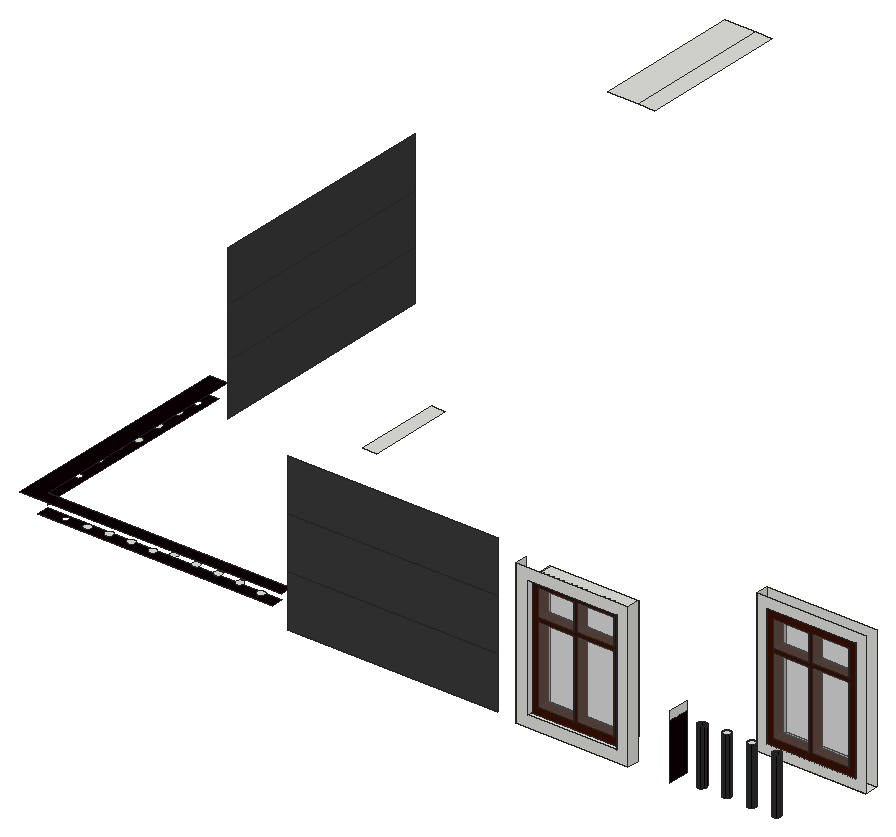
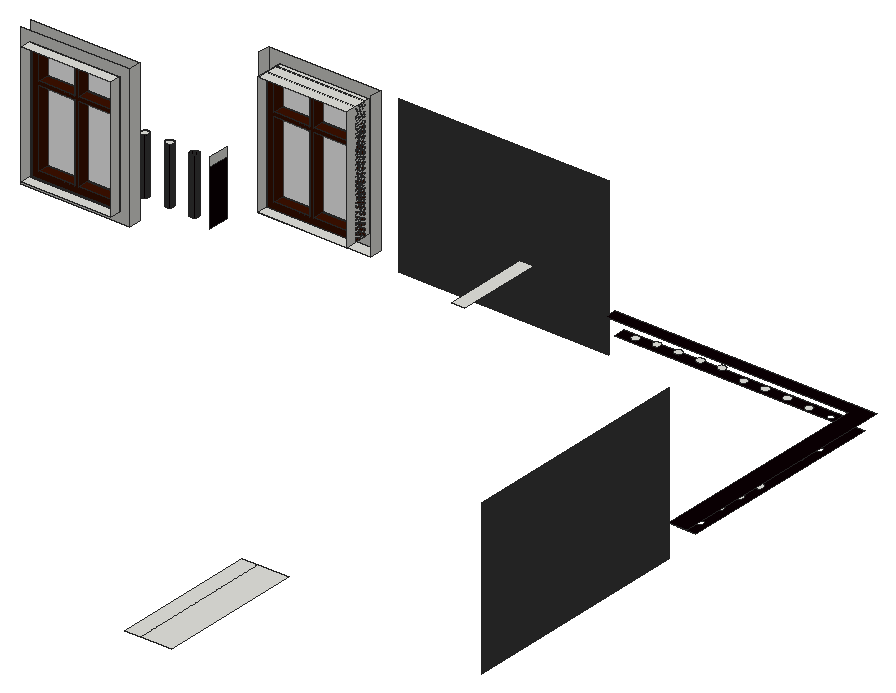
# SketchUp Ruby script. Lengths in inches.
U = 1.inch
M = Sketchup.active_model
def pt(a) = Geom::Point3d.new(a.map { |v| v * U })
def face(e, loops, mat)
  f = e.add_face(loops[0].map { |a| pt(a) })
  loops[1..].each { |l| e.add_face(l.map { |a| pt(a) }).erase! }
  f.material = f.back_material = mat if mat
  f
end
# faces: each face lists its corners as indices into pts; further lists are holes
def faces(e, pts, list, mat = nil) = list.each { |f| face(e, (f[0].is_a?(Array) ? f : [f]).map { |l| l.map { |i| pts[i] } }, mat) }
# xy, xz, yz: faces in a plane at the given z, y or x. An outline is a flat list of corners, or four numbers for a rectangle; further outlines are holes
def ring(l) = l.size == 4 ? [[l[0], l[1]], [l[2], l[1]], [l[2], l[3]], [l[0], l[3]]] : l.each_slice(2).to_a
def flat(e, list, mat, &to3) = list.each { |f| face(e, (f[0].is_a?(Array) ? f : [f]).map { |l| ring(l).map { |u, v| to3.(u, v) } }, mat) }
def xy(e, z, list, mat = nil) = flat(e, list, mat) { |x, y| [x, y, z] }
def xz(e, y, list, mat = nil) = flat(e, list, mat) { |x, z| [x, y, z] }
def yz(e, x, list, mat = nil) = flat(e, list, mat) { |y, z| [x, y, z] }
def lines(e, pts, list) = list.each { |a, b| e.add_line(pt(pts[a]), pt(pts[b])) }
# prism: a flat outline (further loops are holes) pulled along v
def prism(e, loops, v, mat = nil)
  f = face(e, loops, mat); d = Geom::Vector3d.new(v.map { |x| x * U })
  f.pushpull(f.normal.samedirection?(d) ? d.length : -d.length)
end
def box(e, o, s, mat = nil) = prism(e, [[o, [o[0] + s[0], o[1], o[2]], [o[0] + s[0], o[1] + s[1], o[2]], [o[0], o[1] + s[1], o[2]]]], [0, 0, s[2]], mat)
def at(x, y, z, deg = 0) = Geom::Transformation.translation(pt([x, y, z])) * Geom::Transformation.rotation(ORIGIN, Z_AXIS, deg.degrees)
def axes(o, x, y, z) = Geom::Transformation.new([*x, 0, *y, 0, *z, 0, *pt(o).to_a, 1])
def part(name) = M.definitions.add(name)
# library, detail: a bought-in or finely detailed component or shape, given as its bounding box
def library(name, o, s) = part(name).tap { |d| box(d.entities, o, s) }
def detail(e, o, s) = box(e.add_group.entities, o, s)
def put(e, d, t, mat = nil) = e.add_instance(d, t).tap { |i| i.material = mat if mat }
def group(e, t, mat = nil) = e.add_group.tap { |g| g.transformation = t; g.material = mat if mat }.entities
root = M.entities
M.materials.add("[Color C08]").color = [60, 17, 0]
M.materials.add("[Color M07]").color = [58, 58, 58]
M.materials.add("[Metal Seamed]").color = [11, 0, 4]
M.materials.add("[Translucent Glass Gray]").color = [128, 128, 128]
M.materials["[Translucent Glass Gray]"].alpha = 0.5
c1 = part("Group\#3")
xy(c1.entities,0,[[0,0,51.6875,4]],"[Color C08]")
xy(c1.entities,4.05,[[4.05,0,24.41,4],[24.41,0,26.55,4],[26.55,0,47.64,4]],"[Color C08]")
xy(c1.entities,49.59,[[4.05,0,24.41,4],[26.55,0,47.64,4]],"[Color C08]")
xy(c1.entities,51.6875,[[4.05,0,24.41,4],[26.55,0,47.64,4]],"[Color C08]")
xy(c1.entities,67.57,[[4.05,0,24.41,4],[26.55,0,47.64,4]],"[Color C08]")
xy(c1.entities,71.625,[[0,0,51.6875,4]],"[Color C08]")
xz(c1.entities,0,[[[0,0,51.6875,71.625],[4.05,4.05,4.05,49.59,24.41,49.59,24.41,4.05,26.55,4.05,26.55,49.59,47.64,49.59,47.64,4.05],[26.55,51.6875,47.64,67.57],[4.05,51.6875,24.41,67.57]]],"[Color C08]")
xz(c1.entities,0,[[4.05,4.05,24.41,49.59],[26.55,4.05,47.64,49.59],[4.05,51.6875,24.41,67.57],[26.55,51.6875,47.64,67.57]],"[Translucent Glass Gray]")
xz(c1.entities,4,[[[0,0,51.6875,71.625],[4.05,4.05,4.05,49.59,24.41,49.59,24.41,4.05,26.55,4.05,26.55,49.59,47.64,49.59,47.64,4.05],[26.55,51.6875,47.64,67.57],[4.05,51.6875,24.41,67.57]]],"[Color C08]")
yz(c1.entities,0,[[0,0,4,71.625]],"[Color C08]")
yz(c1.entities,4.05,[[0,4.05,4,49.59],[0,51.6875,4,67.57]],"[Color C08]")
yz(c1.entities,24.41,[[0,4.05,4,49.59],[0,51.6875,4,67.57]],"[Color C08]")
yz(c1.entities,26.55,[[0,4.05,4,49.59],[0,51.6875,4,67.57]],"[Color C08]")
yz(c1.entities,47.64,[[0,4.05,4,49.59],[0,51.6875,4,67.57]],"[Color C08]")
yz(c1.entities,51.6875,[[0,0,4,71.625]],"[Color C08]")
xy(root,300,[[382.22,74.99,381.61,75.05,381.05,75.25,380.55,75.6,380.16,76.06,379.91,76.61,379.8,77.2,379.85,77.8,380.06,78.37,380.41,78.86,380.87,79.25,381.41,79.51,382.01,79.61,382.61,79.5625,383.18,79.36,383.67,79.01,384.0625,78.55,384.32,78,384.42,77.41,384.37,76.81,384.16,76.24,383.82,75.74,383.36,75.36,382.81,75.1],[396.15,74.99,395.55,75.05,394.98,75.25,394.49,75.6,394.1,76.06,393.85,76.61,393.74,77.2,393.79,77.8,394,78.37,394.34,78.86,394.81,79.25,395.35,79.51,395.95,79.61,396.55,79.5625,397.12,79.36,397.61,79.01,398,78.55,398.25,78,398.36,77.41,398.31,76.81,398.1,76.24,397.76,75.74,397.29,75.36,396.75,75.1],[410.09,74.99,409.49,75.05,408.92,75.25,408.43,75.6,408.04,76.06,407.78,76.61,407.68,77.2,407.73,77.8,407.94,78.37,408.28,78.86,408.74,79.25,409.29,79.51,409.88,79.61,410.49,79.5625,411.05,79.36,411.55,79.01,411.9375,78.55,412.19,78,412.3,77.41,412.25,76.81,412.04,76.24,411.69,75.74,411.23,75.36,410.69,75.1],[424.03,74.99,423.43,75.05,422.86,75.25,422.36,75.6,421.98,76.06,421.72,76.61,421.61,77.2,421.67,77.8,421.87,78.37,422.22,78.86,422.68,79.25,423.23,79.51,423.82,79.61,424.42,79.5625,424.99,79.36,425.49,79.01,425.875,78.55,426.13,78,426.24,77.41,426.18,76.81,425.98,76.24,425.63,75.74,425.17,75.36,424.62,75.1]])
xy(root,306.73,[[291.14,60.85,353.83,67.28]])
xy(root,307.48,[[389.45,106.41,450.64,113.66]])
xy(root,313.04,[[297.45,60.85,347.52,76.28],[395.02,106.41,445.08,113.66],[395.02,113.66,445.08,119.66]])
xy(root,316.34,[[[21.75,62.76,153.04,69.57],[33.7,65.03,34.2,65.05,34.6875,65.21,35.11,65.48,35.45,65.86,35.68,66.3125,35.78,66.81,35.76,67.3125,35.6,67.79,35.32,68.22,34.95,68.55,34.5,68.78,34,68.89,33.5,68.86,33.02,68.71,32.59,68.43,32.25,68.05,32.02,67.6,31.92,67.11,31.95,66.6,32.1,66.12,32.38,65.7,32.75,65.36,33.21,65.13]]],"[Metal Seamed]")
xy(root,316.6875,[[45.89,65.03,46.39,65.05,46.875,65.21,47.3,65.48,47.64,65.86,47.86,66.3125,47.97,66.81,47.94,67.3125,47.79,67.79,47.51,68.22,47.13,68.55,46.68,68.78,46.1875,68.89,45.68,68.86,45.2,68.71,44.78,68.43,44.44,68.05,44.21,67.6,44.11,67.11,44.13,66.6,44.29,66.12,44.57,65.7,44.94,65.36,45.39,65.13]])
xy(root,317.375,[[58.07,65.03,58.58,65.05,59.0625,65.21,59.48,65.48,59.82,65.86,60.05,66.3125,60.16,66.81,60.13,67.3125,59.97,67.79,59.7,68.22,59.32,68.55,58.87,68.78,58.375,68.89,57.87,68.86,57.39,68.71,56.97,68.43,56.63,68.05,56.4,67.6,56.29,67.11,56.32,66.6,56.48,66.12,56.75,65.7,57.13,65.36,57.58,65.13]])
xy(root,317.4375,[[82.45,65.03,82.95,65.05,83.4375,65.21,83.86,65.48,84.2,65.86,84.43,66.3125,84.53,66.81,84.51,67.3125,84.35,67.79,84.07,68.22,83.7,68.55,83.25,68.78,82.75,68.89,82.25,68.86,81.77,68.71,81.34,68.43,81,68.05,80.77,67.6,80.67,67.11,80.7,66.6,80.85,66.12,81.13,65.7,81.5,65.36,81.96,65.13]])
xy(root,317.5,[[143.07,65.03,143.58,65.05,144.0625,65.21,144.48,65.48,144.82,65.86,145.05,66.3125,145.16,66.81,145.13,67.3125,144.97,67.79,144.7,68.22,144.32,68.55,143.87,68.78,143.375,68.89,142.87,68.86,142.39,68.71,141.97,68.43,141.63,68.05,141.4,67.6,141.29,67.11,141.32,66.6,141.48,66.12,141.75,65.7,142.13,65.36,142.58,65.13]])
xy(root,317.6875,[[70.26,65.03,70.77,65.05,71.25,65.21,71.67,65.48,72.01,65.86,72.24,66.3125,72.34,66.81,72.32,67.3125,72.16,67.79,71.89,68.22,71.51,68.55,71.06,68.78,70.5625,68.89,70.06,68.86,69.58,68.71,69.15,68.43,68.82,68.05,68.59,67.6,68.48,67.11,68.51,66.6,68.66,66.12,68.94,65.7,69.32,65.36,69.77,65.13]])
xy(root,318.625,[[131.2,65.03,131.7,65.05,132.1875,65.21,132.61,65.48,132.95,65.86,133.18,66.3125,133.28,66.81,133.26,67.3125,133.1,67.79,132.82,68.22,132.45,68.55,132,68.78,131.5,68.89,131,68.86,130.52,68.71,130.09,68.43,129.75,68.05,129.52,67.6,129.42,67.11,129.45,66.6,129.6,66.12,129.88,65.7,130.25,65.36,130.71,65.13]])
xy(root,318.9375,[[119.01,65.03,119.52,65.05,120,65.21,120.42,65.48,120.76,65.86,120.99,66.3125,121.09,66.81,121.07,67.3125,120.91,67.79,120.64,68.22,120.26,68.55,119.81,68.78,119.3125,68.89,118.81,68.86,118.33,68.71,117.9,68.43,117.57,68.05,117.34,67.6,117.23,67.11,117.26,66.6,117.41,66.12,117.69,65.7,118.07,65.36,118.52,65.13]])
xy(root,318.96,[[[11.6875,71.13,21.75,188.88],[16.88,177.64,17.49,177.68,18.05,177.88,18.55,178.22,18.95,178.68,19.21,179.22,19.32,179.82,19.28,180.42,19.08,180.99,18.74,181.49,18.28,181.88,17.74,182.14,17.14,182.26,16.54,182.21,15.97,182.01,15.47,181.67,15.08,181.21,14.82,180.67,14.7,180.08,14.75,179.48,14.95,178.91,15.29,178.41,15.75,178.01,16.29,177.75],[16.88,94.39,17.49,94.43,18.05,94.63,18.55,94.97,18.95,95.43,19.21,95.97,19.32,96.57,19.28,97.17,19.08,97.74,18.74,98.24,18.28,98.63,17.74,98.89,17.14,99.01,16.54,98.96,15.97,98.76,15.47,98.42,15.08,97.96,14.82,97.42,14.7,96.83,14.75,96.23,14.95,95.66,15.29,95.16,15.75,94.76,16.29,94.5]]],"[Metal Seamed]")
xy(root,319,[[16.88,136.01,17.49,136.06,18.05,136.26,18.55,136.6,18.95,137.05,19.21,137.6,19.32,138.19,19.28,138.79,19.08,139.36,18.74,139.86,18.28,140.26,17.74,140.52,17.14,140.63,16.54,140.59,15.97,140.39,15.47,140.05,15.08,139.59,14.82,139.05,14.7,138.45,14.75,137.85,14.95,137.28,15.29,136.78,15.75,136.39,16.29,136.125]])
xy(root,319.125,[[106.82,65.03,107.33,65.05,107.8125,65.21,108.23,65.48,108.57,65.86,108.8,66.3125,108.91,66.81,108.88,67.3125,108.72,67.79,108.45,68.22,108.07,68.55,107.62,68.78,107.125,68.89,106.62,68.86,106.14,68.71,105.72,68.43,105.38,68.05,105.15,67.6,105.04,67.11,105.07,66.6,105.23,66.12,105.5,65.7,105.88,65.36,106.33,65.13]])
xy(root,319.8125,[[94.64,65.03,95.14,65.05,95.625,65.21,96.05,65.48,96.39,65.86,96.61,66.3125,96.72,66.81,96.69,67.3125,96.54,67.79,96.26,68.22,95.88,68.55,95.43,68.78,94.9375,68.89,94.43,68.86,93.95,68.71,93.53,68.43,93.19,68.05,92.96,67.6,92.86,67.11,92.88,66.6,93.04,66.12,93.32,65.7,93.69,65.36,94.14,65.13]])
xy(root,319.9375,[[16.88,149.89,17.49,149.93,18.05,150.13,18.55,150.47,18.95,150.93,19.21,151.47,19.32,152.07,19.28,152.67,19.08,153.24,18.74,153.74,18.28,154.13,17.74,154.39,17.14,154.51,16.54,154.46,15.97,154.26,15.47,153.92,15.08,153.46,14.82,152.92,14.7,152.33,14.75,151.73,14.95,151.16,15.29,150.66,15.75,150.26,16.29,150]])
xy(root,320.25,[[16.88,163.76,17.49,163.81,18.05,164.01,18.55,164.35,18.95,164.8,19.21,165.35,19.32,165.94,19.28,166.54,19.08,167.11,18.74,167.61,18.28,168.01,17.74,168.27,17.14,168.38,16.54,168.34,15.97,168.14,15.47,167.8,15.08,167.34,14.82,166.8,14.7,166.2,14.75,165.6,14.95,165.03,15.29,164.53,15.75,164.14,16.29,163.875]])
xy(root,320.875,[[16.88,108.26,17.49,108.31,18.05,108.51,18.55,108.85,18.95,109.3,19.21,109.85,19.32,110.44,19.28,111.04,19.08,111.61,18.74,112.11,18.28,112.51,17.74,112.77,17.14,112.88,16.54,112.84,15.97,112.64,15.47,112.3,15.08,111.84,14.82,111.3,14.7,110.7,14.75,110.1,14.95,109.53,15.29,109.03,15.75,108.64,16.29,108.375]])
xy(root,321.3125,[[16.88,122.14,17.49,122.18,18.05,122.38,18.55,122.72,18.95,123.18,19.21,123.72,19.32,124.32,19.28,124.92,19.08,125.49,18.74,125.99,18.28,126.38,17.74,126.64,17.14,126.76,16.54,126.71,15.97,126.51,15.47,126.17,15.08,125.71,14.82,125.17,14.7,124.58,14.75,123.98,14.95,123.41,15.29,122.91,15.75,122.51,16.29,122.25]])
xy(root,322.6875,[[16.88,80.51,17.49,80.56,18.05,80.76,18.55,81.1,18.95,81.55,19.21,82.1,19.32,82.69,19.28,83.29,19.08,83.86,18.74,84.36,18.28,84.76,17.74,85.02,17.14,85.13,16.54,85.09,15.97,84.89,15.47,84.55,15.08,84.09,14.82,83.55,14.7,82.95,14.75,82.35,14.95,81.78,15.29,81.28,15.75,80.89,16.29,80.625]])
xy(root,324,[[11.6875,62.76,158,62.76,158,69.57,21.75,69.57,21.75,195.41,11.6875,195.41]],"[Metal Seamed]")
xy(root,331.5,[[410.09,74.99,410.69,75.1,411.23,75.36,411.69,75.74,412.04,76.24,412.25,76.81,412.3,77.41,412.19,78,411.9375,78.55,411.55,79.01,411.05,79.36,410.49,79.5625,409.88,79.61,409.29,79.51,408.74,79.25,408.28,78.86,407.94,78.37,407.73,77.8,407.68,77.2,407.78,76.61,408.04,76.06,408.43,75.6,408.92,75.25,409.49,75.05]])
xy(root,331.625,[[396.15,74.99,396.75,75.1,397.29,75.36,397.76,75.74,398.1,76.24,398.31,76.81,398.36,77.41,398.25,78,398,78.55,397.61,79.01,397.12,79.36,396.55,79.5625,395.95,79.61,395.35,79.51,394.81,79.25,394.34,78.86,394,78.37,393.79,77.8,393.74,77.2,393.85,76.61,394.1,76.06,394.49,75.6,394.98,75.25,395.55,75.05]])
xy(root,372,[[158,120.11,165.5625,168.11]])
xy(root,380.98,[[297.45,60.85,347.52,76.28],[395.02,106.41,445.08,113.66],[395.02,113.66,445.08,119.66]])
xy(root,383.34,[[55.1875,419.61,72.6875,501.8],[72.6875,419.61,81.6875,501.8]])
xz(root,60.85,[[[291.14,306.73,353.83,387.29],[297.45,313.04,347.52,380.98]]])
xz(root,67.28,[[158,304.25,275.92,333.3125],[158,333.3125,275.92,362.375],[158,362.375,275.92,391.4375]],"[Color M07]")
xz(root,106.41,[[[389.45,307.48,450.64,386.54],[395.02,313.04,445.08,380.98]]])
xz(root,113.66,[[[389.45,307.48,450.64,386.54],[395.02,313.04,445.08,380.98]]])
yz(root,21.75,[[69.57,317.84,71.13,320.52]])
yz(root,21.75,[[195.41,305.78,326.53,334.34],[195.41,334.34,326.53,362.9],[195.41,362.9,326.53,391.47]],"[Color M07]")
yz(root,291.14,[[60.85,306.73,67.28,387.29]])
yz(root,297.45,[[60.85,313.04,76.28,380.98]])
yz(root,347.52,[[60.85,313.04,76.28,380.98]])
yz(root,353.83,[[60.85,306.73,67.28,387.29]])
yz(root,369.3125,[[70.97,331.08,82.57,336]])
yz(root,369.3125,[[70.97,300,82.57,331.08]],"[Metal Seamed]")
yz(root,389.45,[[106.41,307.48,113.66,386.54]])
yz(root,395.02,[[106.41,313.04,113.66,380.98],[113.66,313.04,119.66,380.98]])
p = [[381.05,75.25,300],[381.61,75.05,300],[381.61,75.05,331.08],[381.05,75.25,331.08],[382.22,74.99,300],[382.22,74.99,331.08],
  [382.81,75.1,300],[382.81,75.1,331.08],[394.98,75.25,300],[395.55,75.05,300],[395.55,75.05,331.625],[394.98,75.25,331.625],
  [396.15,74.99,300],[396.15,74.99,331.625],[396.75,75.1,300],[396.75,75.1,331.625],[408.92,75.25,300],[409.49,75.05,300],
  [409.49,75.05,331.5],[408.92,75.25,331.5],[410.09,74.99,300],[410.09,74.99,331.5],[410.69,75.1,300],[410.69,75.1,331.5],
  [422.86,75.25,300],[423.43,75.05,300],[423.43,75.05,331.08],[422.86,75.25,331.08],[424.03,74.99,300],[424.03,74.99,331.08],
  [424.62,75.1,300],[424.62,75.1,331.08],[383.36,75.36,300],[383.36,75.36,331.08],[397.29,75.36,300],[397.29,75.36,331.625],
  [411.23,75.36,300],[411.23,75.36,331.5],[425.17,75.36,300],[425.17,75.36,331.08],[380.55,75.6,300],[380.55,75.6,331.08],
  [394.49,75.6,300],[394.49,75.6,331.625],[408.43,75.6,300],[408.43,75.6,331.5],[422.36,75.6,300],[422.36,75.6,331.08],
  [383.82,75.74,300],[383.82,75.74,331.08],[397.76,75.74,300],[397.76,75.74,331.625],[411.69,75.74,300],[411.69,75.74,331.5],
  [425.63,75.74,300],[425.63,75.74,331.08],[380.16,76.06,300],[380.16,76.06,331.08],[394.1,76.06,300],[394.1,76.06,331.625],
  [408.04,76.06,300],[408.04,76.06,331.5],[421.98,76.06,300],[421.98,76.06,331.08],[384.16,76.24,300],[384.16,76.24,331.08],
  [398.1,76.24,300],[398.1,76.24,331.625],[412.04,76.24,300],[412.04,76.24,331.5],[425.98,76.24,300],[425.98,76.24,331.08],
  [379.91,76.61,300],[379.91,76.61,331.08],[393.85,76.61,300],[393.85,76.61,331.625],[407.78,76.61,300],[407.78,76.61,331.5],
  [421.72,76.61,300],[421.72,76.61,331.08],[384.37,76.81,300],[384.37,76.81,331.08],[398.31,76.81,300],[398.31,76.81,331.625],
  [412.25,76.81,300],[412.25,76.81,331.5],[426.18,76.81,300],[426.18,76.81,331.08],[379.8,77.2,300],[379.8,77.2,331.08],
  [393.74,77.2,300],[393.74,77.2,331.625],[407.68,77.2,300],[407.68,77.2,331.5],[421.61,77.2,300],[421.61,77.2,331.08],
  [384.42,77.41,300],[384.42,77.41,331.08],[398.36,77.41,300],[398.36,77.41,331.625],[412.3,77.41,300],[412.3,77.41,331.5],
  [426.24,77.41,300],[426.24,77.41,331.08],[379.85,77.8,300],[379.85,77.8,331.08],[393.79,77.8,300],[393.79,77.8,331.625],
  [407.73,77.8,300],[407.73,77.8,331.5],[421.67,77.8,300],[421.67,77.8,331.08],[384.32,78,300],[384.32,78,331.08],
  [398.25,78,300],[398.25,78,331.625],[412.19,78,300],[412.19,78,331.5],[426.13,78,300],[426.13,78,331.08],
  [380.06,78.37,300],[380.06,78.37,331.08],[394,78.37,300],[394,78.37,331.625],[407.94,78.37,300],[407.94,78.37,331.5],
  [421.87,78.37,300],[421.87,78.37,331.08],[384.0625,78.55,300],[384.0625,78.55,331.08],[398,78.55,300],[398,78.55,331.625],
  [411.9375,78.55,300],[411.9375,78.55,331.5],[425.875,78.55,300],[425.875,78.55,331.08],[380.41,78.86,300],[380.41,78.86,331.08],
  [394.34,78.86,300],[394.34,78.86,331.625],[408.28,78.86,300],[408.28,78.86,331.5],[422.22,78.86,300],[422.22,78.86,331.08],
  [383.67,79.01,300],[383.67,79.01,331.08],[397.61,79.01,300],[397.61,79.01,331.625],[411.55,79.01,300],[411.55,79.01,331.5],
  [425.49,79.01,300],[425.49,79.01,331.08],[380.87,79.25,300],[380.87,79.25,331.08],[394.81,79.25,300],[394.81,79.25,331.625],
  [408.74,79.25,300],[408.74,79.25,331.5],[422.68,79.25,300],[422.68,79.25,331.08],[383.18,79.36,300],[383.18,79.36,331.08],
  [397.12,79.36,300],[397.12,79.36,331.625],[411.05,79.36,300],[411.05,79.36,331.5],[424.99,79.36,300],[424.99,79.36,331.08],
  [381.41,79.51,300],[381.41,79.51,331.08],[395.35,79.51,300],[395.35,79.51,331.625],[409.29,79.51,300],[409.29,79.51,331.5],
  [423.23,79.51,300],[423.23,79.51,331.08],[382.61,79.5625,300],[382.61,79.5625,331.08],[396.55,79.5625,300],[396.55,79.5625,331.625],
  [410.49,79.5625,300],[410.49,79.5625,331.5],[424.42,79.5625,300],[424.42,79.5625,331.08],[382.01,79.61,300],[382.01,79.61,331.08],
  [395.95,79.61,300],[395.95,79.61,331.625],[409.88,79.61,300],[409.88,79.61,331.5],[423.82,79.61,300],[423.82,79.61,331.08]]
faces(root,p,[[0,1,2,3],[1,4,5,2],[4,6,7,5],[8,9,10,11],[9,12,13,10],[12,14,15,13],[16,17,18,19],[17,20,21,18],
  [20,22,23,21],[24,25,26,27],[25,28,29,26],[28,30,31,29],[6,32,33,7],[14,34,35,15],[22,36,37,23],[30,38,39,31],
  [40,0,3,41],[42,8,11,43],[44,16,19,45],[46,24,27,47],[32,48,49,33],[34,50,51,35],[36,52,53,37],[38,54,55,39],
  [56,40,41,57],[58,42,43,59],[60,44,45,61],[62,46,47,63],[48,64,65,49],[50,66,67,51],[52,68,69,53],[54,70,71,55],
  [72,56,57,73],[74,58,59,75],[76,60,61,77],[78,62,63,79],[64,80,81,65],[66,82,83,67],[68,84,85,69],[70,86,87,71],
  [88,72,73,89],[90,74,75,91],[92,76,77,93],[94,78,79,95],[80,96,97,81],[82,98,99,83],[84,100,101,85],[86,102,103,87],
  [104,88,89,105],[106,90,91,107],[108,92,93,109],[110,94,95,111],[96,112,113,97],[98,114,115,99],[100,116,117,101],[102,118,119,103],
  [120,104,105,121],[122,106,107,123],[124,108,109,125],[126,110,111,127],[112,128,129,113],[114,130,131,115],[116,132,133,117],[118,134,135,119],
  [136,120,121,137],[138,122,123,139],[140,124,125,141],[142,126,127,143],[128,144,145,129],[130,146,147,131],[132,148,149,133],[134,150,151,135],
  [152,136,137,153],[154,138,139,155],[156,140,141,157],[158,142,143,159],[144,160,161,145],[146,162,163,147],[148,164,165,149],[150,166,167,151],
  [168,152,153,169],[170,154,155,171],[172,156,157,173],[174,158,159,175],[160,176,177,161],[162,178,179,163],[164,180,181,165],[166,182,183,167],
  [184,168,169,185],[186,170,171,187],[188,172,173,189],[190,174,175,191],[176,184,185,177],[178,186,187,179],[180,188,189,181],[182,190,191,183]],"[Metal Seamed]")
put(root,c1,axes([297.45,63.78,313.04],[0.96856,0,0],[0,1.6104,0],[0,0,0.94852]))
put(root,c1,axes([395.02,106.41,313.04],[0.96856,0,0],[0,1.6104,0],[0,0,0.94852]))
